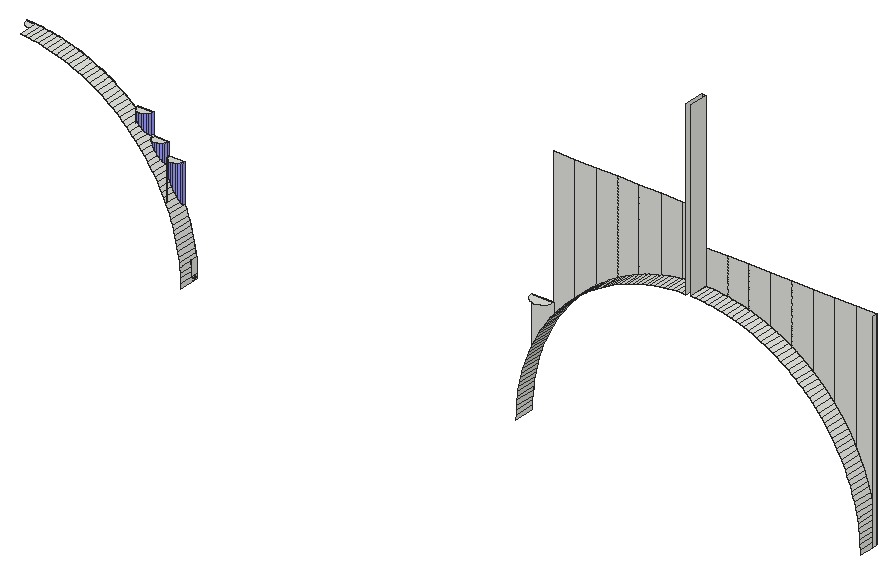
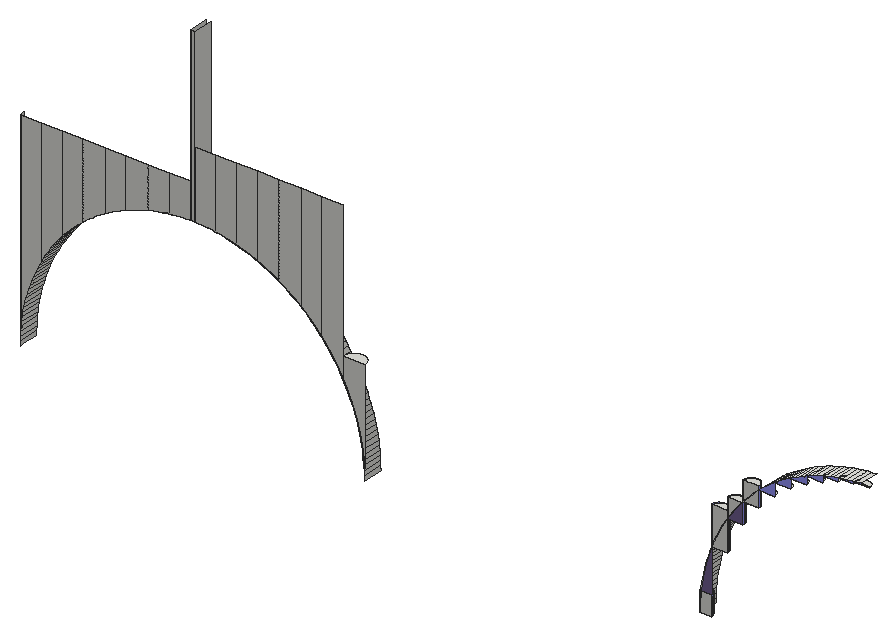
# SketchUp Ruby script. Lengths in inches.
U = 1.inch
M = Sketchup.active_model
def pt(a) = Geom::Point3d.new(a.map { |v| v * U })
def face(e, loops, mat)
  f = e.add_face(loops[0].map { |a| pt(a) })
  loops[1..].each { |l| e.add_face(l.map { |a| pt(a) }).erase! }
  f.material = f.back_material = mat if mat
  f
end
# faces: each face lists its corners as indices into pts; further lists are holes
def faces(e, pts, list, mat = nil) = list.each { |f| face(e, (f[0].is_a?(Array) ? f : [f]).map { |l| l.map { |i| pts[i] } }, mat) }
# xy, xz, yz: faces in a plane at the given z, y or x. An outline is a flat list of corners, or four numbers for a rectangle; further outlines are holes
def ring(l) = l.size == 4 ? [[l[0], l[1]], [l[2], l[1]], [l[2], l[3]], [l[0], l[3]]] : l.each_slice(2).to_a
def flat(e, list, mat, &to3) = list.each { |f| face(e, (f[0].is_a?(Array) ? f : [f]).map { |l| ring(l).map { |u, v| to3.(u, v) } }, mat) }
def xy(e, z, list, mat = nil) = flat(e, list, mat) { |x, y| [x, y, z] }
def xz(e, y, list, mat = nil) = flat(e, list, mat) { |x, z| [x, y, z] }
def yz(e, x, list, mat = nil) = flat(e, list, mat) { |y, z| [x, y, z] }
def lines(e, pts, list) = list.each { |a, b| e.add_line(pt(pts[a]), pt(pts[b])) }
# prism: a flat outline (further loops are holes) pulled along v
def prism(e, loops, v, mat = nil)
  f = face(e, loops, mat); d = Geom::Vector3d.new(v.map { |x| x * U })
  f.pushpull(f.normal.samedirection?(d) ? d.length : -d.length)
end
def box(e, o, s, mat = nil) = prism(e, [[o, [o[0] + s[0], o[1], o[2]], [o[0] + s[0], o[1] + s[1], o[2]], [o[0], o[1] + s[1], o[2]]]], [0, 0, s[2]], mat)
def at(x, y, z, deg = 0) = Geom::Transformation.translation(pt([x, y, z])) * Geom::Transformation.rotation(ORIGIN, Z_AXIS, deg.degrees)
def axes(o, x, y, z) = Geom::Transformation.new([*x, 0, *y, 0, *z, 0, *pt(o).to_a, 1])
def part(name) = M.definitions.add(name)
# library, detail: a bought-in or finely detailed component or shape, given as its bounding box
def library(name, o, s) = part(name).tap { |d| box(d.entities, o, s) }
def detail(e, o, s) = box(e.add_group.entities, o, s)
def put(e, d, t, mat = nil) = e.add_instance(d, t).tap { |i| i.material = mat if mat }
def group(e, t, mat = nil) = e.add_group.tap { |g| g.transformation = t; g.material = mat if mat }.entities
root = M.entities
M.materials.add("[Color I01]").color = [116, 98, 147]
M.materials.add("[Color I02]").color = [153, 153, 255]
xy(root,65.41,[[153.458,140.666,153.321,140.684,153.193,140.737,153.083,140.822,152.998,140.932,152.945,141.06,152.927,141.197,153.72,141.197,153.72,140.735,153.596,140.684]])
xy(root,66.722,[[153.458,140.666,153.596,140.684,153.72,140.735,153.72,141.197,152.927,141.197,152.945,141.06,152.998,140.932,153.083,140.822,153.193,140.737,153.321,140.684]])
xy(root,69.616,[[152.396,140.666,152.258,140.684,152.13,140.737,152.02,140.822,151.936,140.932,151.883,141.06,151.864,141.197,152.927,141.197,152.909,141.06,152.856,140.932,152.771,140.822,152.661,140.737,152.533,140.684]])
xy(root,71.69,[[151.333,140.666,151.196,140.684,151.068,140.737,150.958,140.822,150.873,140.932,150.82,141.06,150.802,141.197,151.864,141.197,151.846,141.06,151.793,140.932,151.709,140.822,151.599,140.737,151.471,140.684]])
xy(root,72.179,[[152.396,140.666,152.533,140.684,152.661,140.737,152.771,140.822,152.856,140.932,152.909,141.06,152.927,141.197,151.864,141.197,151.883,141.06,151.936,140.932,152.02,140.822,152.13,140.737,152.258,140.684]])
xy(root,72.397,[[176.942,140.478,177.128,140.503,177.302,140.575,177.451,140.689,177.565,140.838,177.637,141.011,177.661,141.197,176.224,141.197,176.248,141.011,176.32,140.838,176.434,140.689,176.583,140.575,176.756,140.503]])
xy(root,73.003,[[151.333,140.666,151.471,140.684,151.599,140.737,151.709,140.822,151.793,140.932,151.846,141.06,151.864,141.197,150.802,141.197,150.82,141.06,150.873,140.932,150.958,140.822,151.068,140.737,151.196,140.684]])
xy(root,73.087,[[150.271,140.666,150.133,140.684,150.005,140.737,149.895,140.822,149.811,140.932,149.758,141.06,149.739,141.197,150.802,141.197,150.784,141.06,150.731,140.932,150.646,140.822,150.536,140.737,150.408,140.684]])
xy(root,74.138,[[149.208,140.666,149.346,140.684,149.474,140.737,149.584,140.822,149.668,140.932,149.721,141.06,149.739,141.197,148.677,141.197,148.695,141.06,148.748,140.932,148.833,140.822,148.943,140.737,149.071,140.684]])
xy(root,74.399,[[150.271,140.666,150.408,140.684,150.536,140.737,150.646,140.822,150.731,140.932,150.784,141.06,150.802,141.197,149.739,141.197,149.758,141.06,149.811,140.932,149.895,140.822,150.005,140.737,150.133,140.684]])
xy(root,74.958,[[148.146,140.666,148.283,140.684,148.411,140.737,148.521,140.822,148.606,140.932,148.659,141.06,148.677,141.197,147.614,141.197,147.633,141.06,147.686,140.932,147.77,140.822,147.88,140.737,148.008,140.684]])
xy(root,75.603,[[147.083,140.666,147.221,140.684,147.349,140.737,147.459,140.822,147.543,140.932,147.596,141.06,147.614,141.197,146.552,141.197,146.57,141.06,146.623,140.932,146.708,140.822,146.818,140.737,146.946,140.684]])
xy(root,76.103,[[146.021,140.666,146.158,140.684,146.286,140.737,146.396,140.822,146.481,140.932,146.534,141.06,146.552,141.197,145.489,141.197,145.508,141.06,145.561,140.932,145.645,140.822,145.755,140.737,145.883,140.684]])
xy(root,76.481,[[144.958,140.666,145.096,140.684,145.224,140.737,145.334,140.822,145.418,140.932,145.471,141.06,145.489,141.197,144.427,141.197,144.445,141.06,144.498,140.932,144.583,140.822,144.693,140.737,144.821,140.684]])
xy(root,76.747,[[143.896,140.666,144.033,140.684,144.161,140.737,144.271,140.822,144.356,140.932,144.409,141.06,144.427,141.197,143.364,141.197,143.383,141.06,143.436,140.932,143.52,140.822,143.63,140.737,143.758,140.684]])
xy(root,76.908,[[142.833,140.666,142.971,140.684,143.099,140.737,143.209,140.822,143.293,140.932,143.346,141.06,143.364,141.197,142.302,141.197,142.32,141.06,142.373,140.932,142.458,140.822,142.568,140.737,142.696,140.684]])
xy(root,76.971,[[187.931,139.885,187.936,141.197]])
xz(root,141.197,[[152.927,65.41,153.72,65.41,153.716,65.715,153.704,66.02,153.683,66.325,153.655,66.629,153.644,66.722,152.927,66.722],[153.72,65.41,153.716,65.715,153.704,66.02,153.683,66.325,153.655,66.629,153.644,66.722,153.72,66.722],[176.224,65.41,176.224,72.397,177.661,72.397,177.661,70.991,177.601,70.883,177.463,70.617,177.331,70.348,177.206,70.075,177.089,69.798,176.979,69.519,176.876,69.237,176.78,68.953,176.692,68.666,176.611,68.377,176.538,68.086,176.472,67.793,176.414,67.499,176.364,67.203,176.321,66.906,176.286,66.608,176.259,66.309,176.239,66.01,176.228,65.71],[199.349,65.41,199.345,65.715,199.333,66.02,199.3125,66.325,199.284,66.629,199.248,66.932,199.204,67.234,199.152,67.535,199.092,67.834,199.024,68.132,198.948,68.427,198.864,68.721,198.773,69.012,198.674,69.301,198.568,69.587,198.454,69.87,198.332,70.15,198.203,70.427,198.067,70.7,197.993,70.839,197.993,79.3125,199.349,79.3125],[151.864,69.616,151.864,71.69,151.987,71.497,152.145,71.236,152.295,70.97,152.438,70.7,152.574,70.427,152.703,70.15,152.825,69.87,152.927,69.616],
  [152.927,69.616,152.825,69.87,152.703,70.15,152.574,70.427,152.438,70.7,152.295,70.97,152.145,71.236,151.987,71.497,151.864,71.69,151.864,72.179,152.927,72.179],[197.993,70.839,197.924,70.97,197.774,71.236,197.616,71.497,197.452,71.755,197.281,72.008,197.104,72.256,196.92,72.5,196.729,72.738,196.556,72.944,196.556,79.3125,197.993,79.3125],[177.661,70.991,177.661,81.5,179.099,81.5,179.099,73.039,178.949,72.865,178.758,72.634,178.574,72.397,178.395,72.155,178.224,71.909,178.058,71.659,177.899,71.405,177.747,71.146],[151.864,71.69,151.823,71.755,151.652,72.008,151.475,72.256,151.291,72.5,151.1,72.738,150.904,72.972,150.877,73.003,151.864,73.003],[196.556,72.944,196.533,72.972,196.33,73.2,196.121,73.423,195.907,73.64,195.687,73.852,195.461,74.058,195.23,74.257,195.118,74.349,195.118,79.3125,196.556,79.3125],
  [179.099,73.039,179.099,81.5,180.536,81.5,180.536,74.416,180.441,74.34,180.212,74.146,179.988,73.946,179.769,73.741,179.555,73.53,179.347,73.314,179.145,73.092],[149.739,73.087,149.739,74.138,149.832,74.058,150.058,73.852,150.278,73.64,150.492,73.423,150.701,73.2,150.802,73.087],[150.802,73.087,150.701,73.2,150.492,73.423,150.278,73.64,150.058,73.852,149.832,74.058,149.739,74.138,149.739,74.399,150.802,74.399],[195.118,74.349,194.994,74.451,194.753,74.638,194.507,74.818,194.256,74.993,194.001,75.16,193.741,75.321,193.681,75.356,193.681,79.3125,195.118,79.3125],[180.536,74.416,180.536,81.5,181.974,81.5,181.974,75.404,181.915,75.371,181.659,75.215,181.406,75.053,181.158,74.884,180.915,74.709,180.676,74.527],
  [193.681,75.356,193.477,75.474,193.21,75.621,192.938,75.761,192.663,75.893,192.385,76.018,192.243,76.077,192.243,79.3125,193.681,79.3125],[181.974,75.404,181.974,81.5,183.411,81.5,183.411,76.111,183.254,76.047,182.979,75.926,182.708,75.797,182.44,75.662,182.176,75.52],[192.243,76.077,192.103,76.136,191.818,76.246,191.531,76.349,191.241,76.444,190.948,76.531,190.806,76.57,190.806,79.3125,192.243,79.3125],[183.411,76.111,183.411,81.5,184.849,81.5,184.849,76.592,184.669,76.544,184.381,76.459,184.095,76.367,183.812,76.268,183.531,76.161],[190.806,76.57,190.653,76.611,190.357,76.683,190.058,76.747,189.758,76.803,189.457,76.851,189.368,76.863,189.368,79.3125,190.806,79.3125],
  [184.849,76.592,184.849,81.5,186.286,81.5,186.286,76.873,186.136,76.854,185.839,76.807,185.544,76.753,185.25,76.691,184.959,76.621],[189.368,76.863,189.154,76.891,188.85,76.923,188.546,76.947,188.241,76.963,187.936,76.971,187.931,76.971,187.931,79.3125,189.368,79.3125],[186.286,76.873,186.286,81.5,187.631,81.5,187.631,76.952,187.331,76.963,187.031,76.947,186.732,76.924,186.433,76.893],[187.631,76.952,187.931,76.971,187.931,88.4375,187.631,88.4375]])
xz(root,141.197,[[152.927,66.722,153.644,66.722,153.619,66.932,153.575,67.234,153.523,67.535,153.463,67.834,153.395,68.132,153.319,68.427,153.235,68.721,153.144,69.012,153.045,69.301,152.939,69.587,152.927,69.616,152.825,69.87,152.703,70.15,152.574,70.427,152.438,70.7,152.295,70.97,152.145,71.236,151.987,71.497,151.864,71.69,151.823,71.755,151.652,72.008,151.475,72.256,151.291,72.5,151.1,72.738,150.904,72.972,150.877,73.003,150.802,73.003,150.802,71.69,151.864,71.69,151.864,69.616,152.927,69.616]],"[Color I01]")
xz(root,141.197,[[150.802,73.003,150.877,73.003,150.802,73.087,150.701,73.2,150.492,73.423,150.278,73.64,150.058,73.852,149.832,74.058,149.739,74.138,149.601,74.257,149.365,74.451,149.124,74.638,148.878,74.818,148.677,74.958,148.627,74.993,148.372,75.16,148.112,75.321,147.848,75.474,147.614,75.603,147.581,75.621,147.309,75.761,147.034,75.893,146.756,76.018,146.552,76.103,146.474,76.136,146.189,76.246,145.902,76.349,145.612,76.444,145.489,76.481,145.319,76.531,145.024,76.611,144.728,76.683,144.429,76.747,144.427,76.747,144.129,76.803,143.828,76.851,143.525,76.891,143.364,76.908,143.221,76.923,142.917,76.947,142.612,76.963,142.307,76.971,142.302,76.971,142.302,76.908,143.364,76.908,143.364,76.747,144.427,76.747,144.427,76.481,145.489,76.481,145.489,76.103,146.552,76.103,146.552,75.603,147.614,75.603,147.614,74.958,148.677,74.958,148.677,74.138,149.739,74.138,149.739,73.087,150.802,73.087]],"[Color I02]")
yz(root,153.72,[[140.735,65.41,141.197,66.722]])
yz(root,187.631,[[139.885,76.952,141.197,88.4375]])
yz(root,187.931,[[139.885,76.971,141.197,88.4375]])
yz(root,199.349,[[140.872,65.41,141.197,79.3125]])
p = [[153.716,141.197,65.715],[153.72,141.197,65.41],[153.72,140.735,65.41],[153.72,139.885,65.41],[153.716,139.885,65.715],[176.224,141.197,65.41],
  [176.228,141.197,65.71],[176.228,139.885,65.71],[176.224,139.885,65.41],[199.345,141.197,65.715],[199.349,141.197,65.41],[199.349,140.872,65.41],
  [199.349,139.885,65.41],[199.345,139.885,65.715],[153.083,140.822,65.41],[153.193,140.737,65.41],[153.193,140.737,66.722],[153.083,140.822,66.722],
  [153.321,140.684,65.41],[153.321,140.684,66.722],[153.458,140.666,65.41],[153.458,140.666,66.722],[153.596,140.684,65.41],[153.596,140.684,66.722],
  [153.72,140.735,66.722],[152.998,140.932,65.41],[152.998,140.932,66.722],[152.945,141.06,65.41],[152.945,141.06,66.722],[152.927,141.197,65.41],
  [152.927,141.197,66.722],[153.704,141.197,66.02],[153.704,139.885,66.02],[176.239,141.197,66.01],[176.239,139.885,66.01],[199.333,141.197,66.02],
  [199.333,139.885,66.02],[153.683,141.197,66.325],[153.683,139.885,66.325],[176.259,141.197,66.309],[176.259,139.885,66.309],[199.3125,141.197,66.325],
  [199.3125,139.885,66.325],[153.655,141.197,66.629],[153.655,139.885,66.629],[176.286,141.197,66.608],[176.286,139.885,66.608],[199.284,141.197,66.629],
  [199.284,139.885,66.629],[153.619,141.197,66.932],[153.644,141.197,66.722],[153.619,139.885,66.932],[176.321,141.197,66.906],[176.32,140.838,66.906],
  [176.321,139.885,66.906],[199.248,141.197,66.932],[199.248,139.885,66.932],[153.575,141.197,67.234],[153.575,139.885,67.234],[176.364,141.197,67.203],
  [176.364,139.885,67.203],[199.204,141.197,67.234],[199.204,139.885,67.234],[153.523,141.197,67.535],[153.523,139.885,67.535],[176.414,141.197,67.499],
  [176.414,139.885,67.499],[199.152,141.197,67.535],[199.152,139.885,67.535],[153.463,141.197,67.834],[153.463,139.885,67.834],[176.472,141.197,67.793],
  [176.472,139.885,67.793],[199.092,141.197,67.834],[199.092,139.885,67.834],[153.395,141.197,68.132],[153.395,139.885,68.132],[176.538,141.197,68.086],
  [176.538,139.885,68.086],[199.024,141.197,68.132],[199.024,139.885,68.132],[153.319,141.197,68.427],[153.319,139.885,68.427],[176.611,141.197,68.377],
  [176.611,139.885,68.377],[198.948,141.197,68.427],[198.948,139.885,68.427],[153.235,141.197,68.721],[153.235,139.885,68.721],[176.692,141.197,68.666],
  [176.692,139.885,68.666],[198.864,141.197,68.721],[198.864,139.885,68.721],[153.144,141.197,69.012],[153.144,139.885,69.012],[176.78,141.197,68.953],
  [176.78,139.885,68.953],[198.773,141.197,69.012],[198.773,139.885,69.012],[153.045,141.197,69.301],[153.045,139.885,69.301],[176.876,141.197,69.237],
  [176.876,139.885,69.237],[198.674,141.197,69.301],[198.674,139.885,69.301],[176.979,141.197,69.519],[176.979,139.885,69.519],[152.939,141.197,69.587],
  [152.939,139.885,69.587],[198.568,141.197,69.587],[198.568,139.885,69.587],[177.089,141.197,69.798],[177.089,139.885,69.798],[152.825,141.197,69.87],
  [152.927,141.197,69.616],[152.825,139.885,69.87],[198.454,141.197,69.87],[198.454,139.885,69.87],[152.02,140.822,69.616],[152.13,140.737,69.616],
  [152.13,140.737,72.179],[152.02,140.822,72.179],[152.258,140.684,69.616],[152.258,140.684,72.179],[152.396,140.666,69.616],[152.396,140.666,72.179],
  [152.533,140.684,69.616],[152.533,140.684,72.179],[152.661,140.737,69.616],[152.661,140.737,72.179],[152.771,140.822,69.616],[152.771,140.822,72.179],
  [151.936,140.932,69.616],[151.936,140.932,72.179],[152.856,140.932,69.616],[152.856,140.932,72.179],[151.883,141.06,69.616],[151.883,141.06,72.179],
  [152.909,141.06,69.616],[152.909,141.06,72.179],[151.864,141.197,69.616],[151.864,141.197,72.179],[151.864,141.197,71.69],[152.927,141.197,72.179],
  [177.206,141.197,70.075],[177.206,139.885,70.075],[152.703,141.197,70.15],[152.703,139.885,70.15],[198.332,141.197,70.15],[198.332,139.885,70.15],
  [177.331,141.197,70.348],[177.331,139.885,70.348],[152.574,141.197,70.427],[152.574,139.885,70.427],[198.203,141.197,70.427],[198.203,139.885,70.427],
  [198.204,140.689,70.427],[177.463,141.197,70.617],[177.463,139.885,70.617],[152.438,141.197,70.7],[152.438,139.885,70.7],[198.067,141.197,70.7],
  [198.067,139.885,70.7],[177.601,141.197,70.883],[177.601,139.885,70.883],[152.295,141.197,70.97],[152.295,139.885,70.97],[197.924,141.197,70.97],
  [197.993,141.197,70.839],[197.924,139.885,70.97],[177.661,141.197,70.991],[177.747,141.197,71.146],[177.747,139.885,71.146],[152.145,141.197,71.236],
  [152.145,139.885,71.236],[197.774,141.197,71.236],[197.774,139.885,71.236],[177.899,141.197,71.405],[177.899,139.885,71.405],[151.987,141.197,71.497],
  [151.987,139.885,71.497],[197.616,141.197,71.497],[197.616,139.885,71.497],[178.058,141.197,71.659],[178.058,139.885,71.659],[151.823,141.197,71.755],
  [151.823,139.885,71.755],[197.452,141.197,71.755],[197.452,139.885,71.755],[178.224,141.197,71.909],[178.224,139.885,71.909],[150.958,140.822,71.69],
  [151.068,140.737,71.69],[151.068,140.737,73.003],[150.958,140.822,73.003],[151.196,140.684,71.69],[151.196,140.684,73.003],[151.333,140.666,71.69],
  [151.333,140.666,73.003],[151.471,140.684,71.69],[151.471,140.684,73.003],[151.599,140.737,71.69],[151.599,140.737,73.003],[151.709,140.822,71.69],
  [151.709,140.822,73.003],[150.873,140.932,71.69],[150.873,140.932,73.003],[151.793,140.932,71.69],[151.793,140.932,73.003],[150.82,141.06,71.69],
  [150.82,141.06,73.003],[151.846,141.06,71.69],[151.846,141.06,73.003],[150.802,141.197,71.69],[150.802,141.197,73.003],[151.864,141.197,73.003],
  [151.652,141.197,72.008],[151.652,139.885,72.008],[197.281,141.197,72.008],[197.281,139.885,72.008],[178.395,141.197,72.155],[178.395,139.885,72.155],
  [151.475,141.197,72.256],[151.475,139.885,72.256],[197.104,141.197,72.256],[197.104,139.885,72.256],[178.574,141.197,72.397],[178.574,139.885,72.397],
  [151.291,141.197,72.5],[151.291,139.885,72.5],[196.92,141.197,72.5],[196.92,139.885,72.5],[178.758,141.197,72.634],[178.758,139.885,72.634],
  [151.1,141.197,72.738],[151.1,139.885,72.738],[196.729,141.197,72.738],[196.729,139.885,72.738],[178.949,141.197,72.865],[178.949,139.885,72.865],
  [150.904,141.197,72.972],[150.904,139.885,72.972],[196.533,141.197,72.972],[196.556,141.197,72.944],[196.533,139.885,72.972],[179.099,141.197,73.039],
  [179.145,141.197,73.092],[179.145,139.885,73.092],[150.701,141.197,73.2],[150.802,141.197,73.087],[150.877,141.197,73.003],[150.701,139.885,73.2],
  [196.33,141.197,73.2],[196.33,139.885,73.2],[179.347,141.197,73.314],[179.347,139.885,73.314],[149.895,140.822,73.087],[150.005,140.737,73.087],
  [150.005,140.737,74.399],[149.895,140.822,74.399],[150.133,140.684,73.087],[150.133,140.684,74.399],[150.271,140.666,73.087],[150.271,140.666,74.399],
  [150.408,140.684,73.087],[150.408,140.684,74.399],[150.536,140.737,73.087],[150.536,140.737,74.399],[150.646,140.822,73.087],[150.646,140.822,74.399],
  [149.811,140.932,73.087],[149.811,140.932,74.399],[150.731,140.932,73.087],[150.731,140.932,74.399],[149.758,141.06,73.087],[149.758,141.06,74.399],
  [150.784,141.06,73.087],[150.784,141.06,74.399],[149.739,141.197,73.087],[149.739,141.197,74.399],[149.739,141.197,74.138],[150.802,141.197,74.399],
  [150.492,141.197,73.423],[150.492,139.885,73.423],[196.121,141.197,73.423],[196.121,139.885,73.423],[179.555,141.197,73.53],[179.555,139.885,73.53],
  [150.278,141.197,73.64],[150.278,139.885,73.64],[195.907,141.197,73.64],[195.907,139.885,73.64],[179.769,141.197,73.741],[179.769,139.885,73.741],
  [150.058,141.197,73.852],[150.058,139.885,73.852],[195.687,141.197,73.852],[195.687,139.885,73.852],[179.988,141.197,73.946],[179.988,139.885,73.946],
  [149.832,141.197,74.058],[149.832,139.885,74.058],[180.212,141.197,74.146],[180.212,139.885,74.146],[195.461,141.197,74.058],[195.461,139.885,74.058],
  [149.601,141.197,74.257],[149.601,139.885,74.257],[180.441,141.197,74.34],[180.441,139.885,74.34],[195.23,141.197,74.257],[195.23,139.885,74.257],
  [149.365,141.197,74.451],[149.365,139.885,74.451],[180.536,141.197,74.416],[180.676,141.197,74.527],[180.676,139.885,74.527],[194.994,141.197,74.451],
  [195.118,141.197,74.349],[194.994,139.885,74.451],[149.124,141.197,74.638],[149.124,139.885,74.638],[180.915,141.197,74.709],[180.915,139.885,74.709],
  [194.753,141.197,74.638],[194.753,139.885,74.638],[148.878,141.197,74.818],[148.878,139.885,74.818],[194.507,141.197,74.818],[194.507,139.885,74.818],
  [181.158,141.197,74.884],[181.158,139.885,74.884],[148.627,141.197,74.993],[148.677,141.197,74.958],[148.627,139.885,74.993],[194.256,141.197,74.993],
  [194.256,139.885,74.993],[181.406,141.197,75.053],[181.406,139.885,75.053],[148.372,141.197,75.16],[148.372,139.885,75.16],[194.001,141.197,75.16],
  [194.001,139.885,75.16],[181.659,141.197,75.215],[181.659,139.885,75.215],[148.112,141.197,75.321],[148.112,139.885,75.321],[181.915,141.197,75.371],
  [181.915,139.885,75.371],[193.741,141.197,75.321],[193.741,139.885,75.321],[147.848,141.197,75.474],[147.848,139.885,75.474],[193.477,141.197,75.474],
  [193.681,141.197,75.356],[193.477,139.885,75.474],[181.974,141.197,75.404],[182.176,141.197,75.52],[182.176,139.885,75.52],[147.581,141.197,75.621],
  [147.614,141.197,75.603],[147.581,139.885,75.621],[182.44,141.197,75.662],[182.44,139.885,75.662],[193.21,141.197,75.621],[193.21,139.885,75.621],
  [147.309,141.197,75.761],[147.309,139.885,75.761],[192.938,141.197,75.761],[192.938,139.885,75.761],[182.708,141.197,75.797],[182.708,139.885,75.797],
  [147.034,141.197,75.893],[147.034,139.885,75.893],[182.979,141.197,75.926],[182.979,139.885,75.926],[192.663,141.197,75.893],[192.663,139.885,75.893],
  [146.756,141.197,76.018],[146.756,139.885,76.018],[183.254,141.197,76.047],[183.254,139.885,76.047],[192.385,141.197,76.018],[192.385,139.885,76.018],
  [146.474,141.197,76.136],[146.552,141.197,76.103],[146.474,139.885,76.136],[183.411,141.197,76.111],[183.531,141.197,76.161],[183.531,139.885,76.161],
  [192.103,141.197,76.136],[192.243,141.197,76.077],[192.103,139.885,76.136],[146.189,141.197,76.246],[146.189,139.885,76.246],[191.818,141.197,76.246],
  [191.818,139.885,76.246],[145.902,141.197,76.349],[145.902,139.885,76.349],[183.812,141.197,76.268],[183.812,139.885,76.268],[191.531,141.197,76.349],
  [191.531,139.885,76.349],[145.612,141.197,76.444],[145.612,139.885,76.444],[184.095,141.197,76.367],[184.095,139.885,76.367],[191.241,141.197,76.444],
  [191.241,139.885,76.444],[145.319,141.197,76.531],[145.489,141.197,76.481],[145.319,139.885,76.531],[184.381,141.197,76.459],[184.381,139.885,76.459],
  [190.948,141.197,76.531],[190.948,139.885,76.531],[145.024,141.197,76.611],[145.024,139.885,76.611],[184.669,141.197,76.544],[184.669,139.885,76.544],
  [184.849,141.197,76.592],[184.959,141.197,76.621],[184.959,139.885,76.621],[190.653,141.197,76.611],[190.806,141.197,76.57],[190.653,139.885,76.611],
  [144.728,141.197,76.683],[144.728,139.885,76.683],[185.25,141.197,76.691],[185.25,139.885,76.691],[190.357,141.197,76.683],[190.357,139.885,76.683],
  [144.129,141.197,76.803],[144.427,141.197,76.747],[144.429,141.197,76.747],[144.429,139.885,76.747],[144.129,139.885,76.803],[185.544,141.197,76.753],
  [185.544,139.885,76.753],[189.758,141.197,76.803],[190.058,141.197,76.747],[190.058,139.885,76.747],[189.758,139.885,76.803],[143.828,141.197,76.851],
  [143.828,139.885,76.851],[185.839,141.197,76.807],[185.839,139.885,76.807],[186.136,141.197,76.854],[186.136,139.885,76.854],[189.457,141.197,76.851],
  [189.457,139.885,76.851],[142.917,141.197,76.947],[143.221,141.197,76.923],[143.221,139.885,76.923],[142.917,139.885,76.947],[143.364,141.197,76.908],
  [143.525,141.197,76.891],[143.525,139.885,76.891],[186.286,141.197,76.873],[186.433,141.197,76.893],[186.433,139.885,76.893],[186.732,141.197,76.924],
  [186.732,139.885,76.924],[187.031,141.197,76.947],[187.031,139.885,76.947],[187.331,141.197,76.963],[187.331,139.885,76.963],[188.241,141.197,76.963],
  [188.546,141.197,76.947],[188.546,139.885,76.947],[188.241,139.885,76.963],[188.85,141.197,76.923],[188.85,139.885,76.923],[189.154,141.197,76.891],
  [189.154,139.885,76.891],[189.368,141.197,76.863],[187.631,141.197,76.952],[187.631,139.885,76.952],[187.936,141.197,76.971],[187.936,139.885,76.971]]
faces(root,p,[[0,1,2,3,4],[5,6,7,8],[9,10,11,12,13],[31,0,4,32],[6,33,34,7],[35,9,13,36],[37,31,32,38],[33,39,40,34],
  [41,35,36,42],[43,37,38,44],[39,45,46,40],[47,41,42,48],[49,50,43,44,51],[45,52,53,54,46],[55,47,48,56],[57,49,51,58],
  [52,59,60,54,53],[61,55,56,62],[63,57,58,64],[59,65,66,60],[67,61,62,68],[69,63,64,70],[65,71,72,66],[73,67,68,74],
  [75,69,70,76],[71,77,78,72],[79,73,74,80],[81,75,76,82],[77,83,84,78],[85,79,80,86],[87,81,82,88],[83,89,90,84],
  [91,85,86,92],[93,87,88,94],[89,95,96,90],[97,91,92,98],[99,93,94,100],[95,101,102,96],[103,97,98,104],[101,105,106,102],
  [107,99,100,108],[109,103,104,110],[105,111,112,106],[113,114,107,108,115],[116,109,110,117],[111,144,145,112],[146,113,115,147],[148,116,117,149],
  [144,150,151,145],[152,146,147,153],[154,148,149,155,156],[150,157,158,151],[159,152,153,160],[161,154,156,155,162],[157,163,164,158],[165,159,160,166],
  [167,168,161,162,169],[163,170,171,172,164],[173,165,166,174],[175,167,169,176],[171,177,178,172],[179,173,174,180],[181,175,176,182],[177,183,184,178],
  [185,142,179,180,186],[187,181,182,188],[183,189,190,184],[216,185,186,217],[218,187,188,219],[189,220,221,190],[222,216,217,223],[224,218,219,225],
  [220,226,227,221],[228,222,223,229],[230,224,225,231],[226,232,233,227],[234,228,229,235],[236,230,231,237],[232,238,239,233],[240,234,235,241],
  [242,243,236,237,244],[238,245,246,247,239],[248,249,250,240,241,251],[252,242,244,253],[246,254,255,247],[282,248,251,283],[284,252,253,285],[254,286,287,255],
  [288,282,283,289],[290,284,285,291],[286,292,293,287],[294,288,289,295],[296,290,291,297],[292,298,299,293],[300,294,295,301],[298,302,303,299],
  [304,296,297,305],[306,280,300,301,307],[302,308,309,303],[310,304,305,311],[312,306,307,313],[308,314,315,316,309],[317,318,310,311,319],[320,312,313,321],
  [315,322,323,316],[324,317,319,325],[326,320,321,327],[328,324,325,329],[322,330,331,323],[332,333,326,327,334],[335,328,329,336],[330,337,338,331],
  [339,332,334,340],[341,335,336,342],[337,343,344,338],[345,339,340,346],[343,347,348,344],[349,341,342,350],[351,345,346,352],[353,354,349,350,355],
  [347,356,357,358,348],[359,360,351,352,361],[357,362,363,358],[364,353,355,365],[366,359,361,367],[368,364,365,369],[362,370,371,363],[372,366,367,373],
  [370,374,375,371],[376,368,369,377],[378,372,373,379],[374,380,381,375],[382,376,377,383],[384,385,378,379,386],[380,387,388,389,381],[390,391,382,383,392],
  [393,384,386,394],[395,390,392,396],[397,393,394,398],[388,399,400,389],[401,395,396,402],[403,397,398,404],[399,405,406,400],[407,401,402,408],
  [409,410,403,404,411],[405,412,413,406],[414,407,408,415],[416,409,411,417],[412,418,419,413],[418,420,421,422,419],[423,424,414,415,425],[426,416,417,427],
  [421,428,429,422],[430,423,425,431],[432,433,434,435,436],[434,426,427,435],[428,437,438,429],[439,440,441,442],[440,430,431,441],[443,432,436,444],
  [437,445,446,438],[445,447,448,446],[449,439,442,450],[451,452,453,454],[452,455,456,457,453],[456,443,444,457],[447,458,459,460,448],[459,461,462,460],
  [461,463,464,462],[463,465,466,464],[467,468,469,470],[468,471,472,469],[471,473,474,472],[473,475,449,450,474],[465,476,477,466],[478,467,470,479]])
faces(root,p,[[14,15,16,17],[15,18,19,16],[18,20,21,19],[20,22,23,21],[22,2,24,23],[25,14,17,26],[27,25,26,28],[29,27,28,30],
  [118,119,120,121],[119,122,123,120],[122,124,125,123],[124,126,127,125],[126,128,129,127],[128,130,131,129],[132,118,121,133],[130,134,135,131],
  [136,132,133,137],[134,138,139,135],[140,136,137,141,142],[138,114,143,139],[191,192,193,194],[192,195,196,193],[195,197,198,196],[197,199,200,198],
  [199,201,202,200],[201,203,204,202],[205,191,194,206],[203,207,208,204],[209,205,206,210],[207,211,212,208],[213,209,210,214],[211,142,141,215,212],
  [256,257,258,259],[257,260,261,258],[260,262,263,261],[262,264,265,263],[264,266,267,265],[266,268,269,267],[270,256,259,271],[268,272,273,269],
  [274,270,271,275],[272,276,277,273],[278,274,275,279,280],[276,249,281,277]],"[Color I02]")
